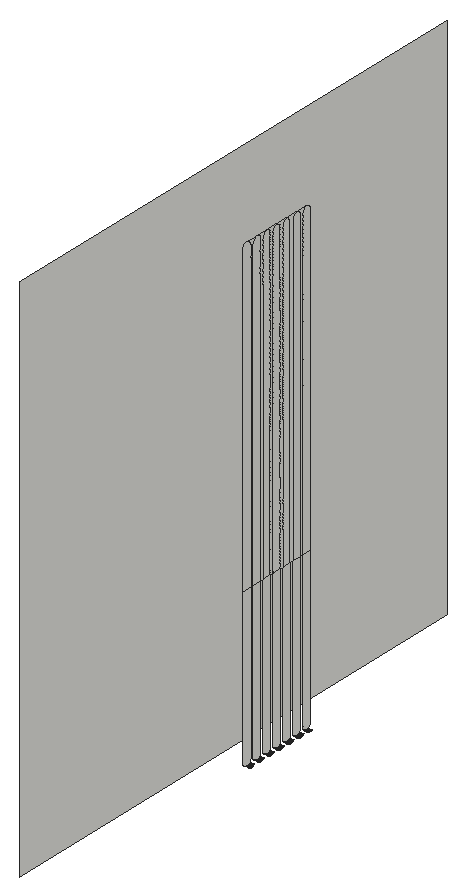
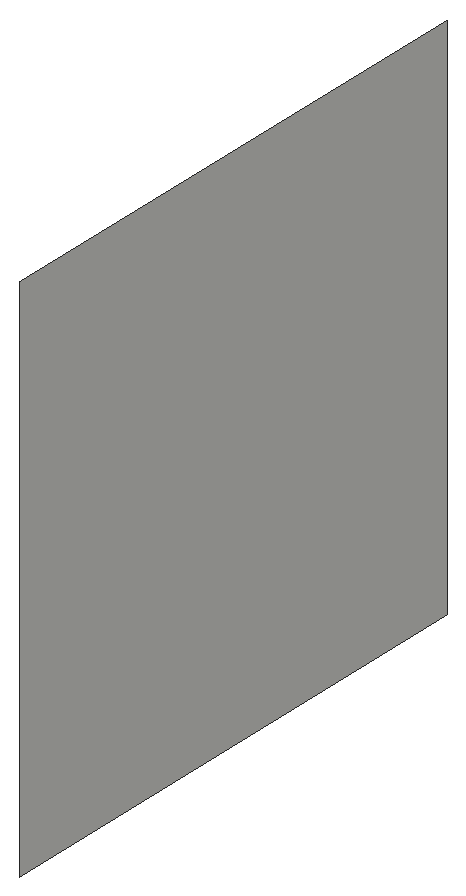
# SketchUp Ruby script. Lengths in inches.
U = 1.inch
M = Sketchup.active_model
def pt(a) = Geom::Point3d.new(a.map { |v| v * U })
def face(e, loops, mat)
  f = e.add_face(loops[0].map { |a| pt(a) })
  loops[1..].each { |l| e.add_face(l.map { |a| pt(a) }).erase! }
  f.material = f.back_material = mat if mat
  f
end
# faces: each face lists its corners as indices into pts; further lists are holes
def faces(e, pts, list, mat = nil) = list.each { |f| face(e, (f[0].is_a?(Array) ? f : [f]).map { |l| l.map { |i| pts[i] } }, mat) }
# xy, xz, yz: faces in a plane at the given z, y or x. An outline is a flat list of corners, or four numbers for a rectangle; further outlines are holes
def ring(l) = l.size == 4 ? [[l[0], l[1]], [l[2], l[1]], [l[2], l[3]], [l[0], l[3]]] : l.each_slice(2).to_a
def flat(e, list, mat, &to3) = list.each { |f| face(e, (f[0].is_a?(Array) ? f : [f]).map { |l| ring(l).map { |u, v| to3.(u, v) } }, mat) }
def xy(e, z, list, mat = nil) = flat(e, list, mat) { |x, y| [x, y, z] }
def xz(e, y, list, mat = nil) = flat(e, list, mat) { |x, z| [x, y, z] }
def yz(e, x, list, mat = nil) = flat(e, list, mat) { |y, z| [x, y, z] }
def lines(e, pts, list) = list.each { |a, b| e.add_line(pt(pts[a]), pt(pts[b])) }
# prism: a flat outline (further loops are holes) pulled along v
def prism(e, loops, v, mat = nil)
  f = face(e, loops, mat); d = Geom::Vector3d.new(v.map { |x| x * U })
  f.pushpull(f.normal.samedirection?(d) ? d.length : -d.length)
end
def box(e, o, s, mat = nil) = prism(e, [[o, [o[0] + s[0], o[1], o[2]], [o[0] + s[0], o[1] + s[1], o[2]], [o[0], o[1] + s[1], o[2]]]], [0, 0, s[2]], mat)
def at(x, y, z, deg = 0) = Geom::Transformation.translation(pt([x, y, z])) * Geom::Transformation.rotation(ORIGIN, Z_AXIS, deg.degrees)
def axes(o, x, y, z) = Geom::Transformation.new([*x, 0, *y, 0, *z, 0, *pt(o).to_a, 1])
def part(name) = M.definitions.add(name)
# library, detail: a bought-in or finely detailed component or shape, given as its bounding box
def library(name, o, s) = part(name).tap { |d| box(d.entities, o, s) }
def detail(e, o, s) = box(e.add_group.entities, o, s)
def put(e, d, t, mat = nil) = e.add_instance(d, t).tap { |i| i.material = mat if mat }
def group(e, t, mat = nil) = e.add_group.tap { |g| g.transformation = t; g.material = mat if mat }.entities
root = M.entities
yz(root,0,[[0,0,120,120]])
yz(root,9,[[52.509,2.396,52.567,2.398,52.624,2.403,52.681,2.41,52.737,2.421,52.792,2.435,52.847,2.452,52.901,2.473,52.954,2.495,53.005,2.521,53.054,2.55,53.103,2.581,53.149,2.615,53.193,2.651,53.235,2.69,53.276,2.731,53.313,2.774,53.349,2.82,53.381,2.867,53.412,2.915,53.439,2.966,53.464,3.018,53.486,3.071,53.504,3.125,53.52,3.18,53.533,3.236,53.543,3.292,53.55,3.363,53.55,38,51.468,38,51.468,3.363,51.476,3.292,51.486,3.236,51.498,3.18,51.514,3.125,51.533,3.071,51.555,3.018,51.579,2.966,51.607,2.915,51.637,2.867,51.67,2.82,51.705,2.774,51.743,2.731,51.783,2.69,51.825,2.651,51.87,2.615,51.916,2.581,51.964,2.55,52.014,2.521,52.065,2.495,52.118,2.473,52.171,2.452,52.226,2.435,52.282,2.421,52.338,2.41,52.395,2.403,52.452,2.398],[55.297,2.396,55.354,2.398,55.411,2.403,55.468,2.41,55.524,2.421,55.58,2.435,55.635,2.452,55.688,2.473,55.741,2.495,55.792,2.521,55.842,2.55,55.89,2.581,55.936,2.615,55.981,2.651,56.023,2.69,56.063,2.731,56.101,2.774,56.136,2.82,56.169,2.867,56.199,2.915,56.227,2.966,56.251,3.018,56.273,3.071,56.292,3.125,56.308,3.18,56.32,3.236,56.33,3.292,56.338,3.363,56.338,38,54.256,38,54.256,3.363,54.263,3.292,54.273,3.236,54.286,3.18,54.302,3.125,54.32,3.071,54.342,3.018,54.367,2.966,54.394,2.915,54.425,2.867,54.457,2.82,54.493,2.774,54.53,2.731,54.571,2.69,54.613,2.651,54.657,2.615,54.703,2.581,54.752,2.55,54.801,2.521,54.852,2.495,54.905,2.473,54.959,2.452,55.014,2.435,55.069,2.421,55.125,2.41,55.182,2.403,55.239,2.398],[58.084,2.396,58.142,2.398,58.199,2.403,58.256,2.41,58.312,2.421,58.367,2.435,58.422,2.452,58.476,2.473,58.529,2.495,58.58,2.521,58.629,2.55,58.678,2.581,58.724,2.615,58.768,2.651,58.81,2.69,58.851,2.731,58.888,2.774,58.924,2.82,58.956,2.867,58.987,2.915,59.014,2.966,59.039,3.018,59.061,3.071,59.079,3.125,59.095,3.18,59.108,3.236,59.118,3.292,59.125,3.363,59.125,38,57.043,38,57.043,3.363,57.051,3.292,57.061,3.236,57.073,3.18,57.089,3.125,57.108,3.071,57.13,3.018,57.154,2.966,57.182,2.915,57.212,2.867,57.245,2.82,57.28,2.774,57.318,2.731,57.358,2.69,57.4,2.651,57.445,2.615,57.491,2.581,57.539,2.55,57.589,2.521,57.64,2.495,57.693,2.473,57.746,2.452,57.801,2.435,57.857,2.421,57.913,2.41,57.97,2.403,58.027,2.398],[60.872,2.396,60.929,2.398,60.986,2.403,61.043,2.41,61.099,2.421,61.155,2.435,61.21,2.452,61.263,2.473,61.316,2.495,61.367,2.521,61.417,2.55,61.465,2.581,61.511,2.615,61.556,2.651,61.598,2.69,61.638,2.731,61.676,2.774,61.711,2.82,61.744,2.867,61.774,2.915,61.802,2.966,61.826,3.018,61.848,3.071,61.867,3.125,61.883,3.18,61.895,3.236,61.905,3.292,61.912,3.363,61.912,38,59.831,38,59.831,3.363,59.838,3.292,59.848,3.236,59.861,3.18,59.877,3.125,59.895,3.071,59.917,3.018,59.942,2.966,59.969,2.915,60,2.867,60.032,2.82,60.068,2.774,60.105,2.731,60.146,2.69,60.188,2.651,60.232,2.615,60.278,2.581,60.327,2.55,60.376,2.521,60.427,2.495,60.48,2.473,60.534,2.452,60.589,2.435,60.644,2.421,60.7,2.41,60.757,2.403,60.814,2.398],[63.659,2.396,63.717,2.398,63.774,2.403,63.831,2.41,63.887,2.421,63.942,2.435,63.997,2.452,64.051,2.473,64.104,2.495,64.155,2.521,64.204,2.55,64.253,2.581,64.299,2.615,64.343,2.651,64.385,2.69,64.426,2.731,64.463,2.774,64.499,2.82,64.531,2.867,64.562,2.915,64.589,2.966,64.614,3.018,64.636,3.071,64.654,3.125,64.67,3.18,64.683,3.236,64.693,3.292,64.7,3.363,64.7,38,62.618,38,62.618,3.363,62.626,3.292,62.636,3.236,62.648,3.18,62.664,3.125,62.683,3.071,62.705,3.018,62.729,2.966,62.757,2.915,62.787,2.867,62.82,2.82,62.855,2.774,62.893,2.731,62.933,2.69,62.975,2.651,63.02,2.615,63.066,2.581,63.114,2.55,63.164,2.521,63.215,2.495,63.268,2.473,63.321,2.452,63.376,2.435,63.432,2.421,63.488,2.41,63.545,2.403,63.602,2.398],
  [66.447,2.396,66.504,2.398,66.561,2.403,66.618,2.41,66.674,2.421,66.73,2.435,66.785,2.452,66.838,2.473,66.891,2.495,66.942,2.521,66.992,2.55,67.04,2.581,67.086,2.615,67.131,2.651,67.173,2.69,67.213,2.731,67.251,2.774,67.286,2.82,67.319,2.867,67.349,2.915,67.377,2.966,67.401,3.018,67.423,3.071,67.442,3.125,67.458,3.18,67.47,3.236,67.48,3.292,67.487,3.363,67.487,38,65.406,38,65.406,3.363,65.413,3.292,65.423,3.236,65.436,3.18,65.452,3.125,65.47,3.071,65.492,3.018,65.517,2.966,65.544,2.915,65.575,2.867,65.607,2.82,65.643,2.774,65.68,2.731,65.721,2.69,65.763,2.651,65.807,2.615,65.853,2.581,65.902,2.55,65.951,2.521,66.002,2.495,66.055,2.473,66.109,2.452,66.164,2.435,66.219,2.421,66.275,2.41,66.332,2.403,66.389,2.398],[69.234,2.396,69.292,2.398,69.349,2.403,69.406,2.41,69.462,2.421,69.517,2.435,69.572,2.452,69.626,2.473,69.679,2.495,69.73,2.521,69.779,2.55,69.828,2.581,69.874,2.615,69.918,2.651,69.96,2.69,70.001,2.731,70.038,2.774,70.074,2.82,70.106,2.867,70.137,2.915,70.164,2.966,70.189,3.018,70.211,3.071,70.229,3.125,70.245,3.18,70.258,3.236,70.268,3.292,70.275,3.363,70.275,38,68.193,38,68.193,3.363,68.201,3.292,68.211,3.236,68.223,3.18,68.239,3.125,68.258,3.071,68.28,3.018,68.304,2.966,68.332,2.915,68.362,2.867,68.395,2.82,68.43,2.774,68.468,2.731,68.508,2.69,68.55,2.651,68.595,2.615,68.641,2.581,68.689,2.55,68.739,2.521,68.79,2.495,68.843,2.473,68.896,2.452,68.951,2.435,69.007,2.421,69.063,2.41,69.12,2.403,69.177,2.398],[53.55,3.363,53.553,3.407,53.553,3.464,53.55,3.521],[54.256,3.363,54.256,3.521,54.253,3.464,54.253,3.407],[56.338,3.363,56.34,3.407,56.34,3.464,56.338,3.521],
  [57.043,3.363,57.043,3.521,57.041,3.464,57.041,3.407],[59.125,3.363,59.128,3.407,59.128,3.464,59.125,3.521],[59.831,3.363,59.831,3.521,59.828,3.464,59.828,3.407],[61.912,3.363,61.915,3.407,61.915,3.464,61.912,3.521],[62.618,3.363,62.618,3.521,62.616,3.464,62.616,3.407],
  [64.7,3.363,64.703,3.407,64.703,3.464,64.7,3.521],[65.406,3.363,65.406,3.521,65.403,3.464,65.403,3.407],[67.487,3.363,67.49,3.407,67.49,3.464,67.487,3.521],[68.193,3.363,68.193,3.521,68.191,3.464,68.191,3.407],[51.468,38,53.55,38,53.55,106.961,53.549,107.015,53.544,107.069,53.537,107.123,53.527,107.177,53.515,107.23,53.499,107.282,53.481,107.334,53.46,107.384,53.437,107.433,53.411,107.481,53.382,107.528,53.351,107.572,53.318,107.616,53.283,107.657,53.245,107.697,53.206,107.734,53.164,107.769,53.121,107.803,53.076,107.834,53.03,107.862,52.982,107.888,52.933,107.911,52.882,107.932,52.831,107.95,52.779,107.966,52.726,107.979,52.672,107.989,52.618,107.996,52.564,108,52.455,108,52.4,107.996,52.346,107.989,52.293,107.979,52.24,107.966,52.1875,107.95,52.136,107.932,52.086,107.911,52.037,107.888,51.989,107.862,51.942,107.834,51.898,107.803,51.854,107.769,51.813,107.734,51.773,107.697,51.736,107.657,51.7,107.616,51.667,107.572,51.636,107.528,51.608,107.481,51.582,107.433,51.558,107.384,51.538,107.334,51.519,107.282,51.504,107.23,51.491,107.177,51.481,107.123,51.474,107.069,51.47,107.015,51.468,106.961],
  [53.55,38,54.256,38,54.256,106.961,54.257,107.015,54.262,107.069,54.269,107.123,54.279,107.177,54.291,107.23,54.307,107.282,54.325,107.334,54.346,107.384,54.369,107.433,54.395,107.481,54.424,107.528,54.455,107.572,54.488,107.616,54.523,107.657,54.561,107.697,54.6,107.734,54.642,107.769,54.685,107.803,54.73,107.834,54.776,107.862,54.824,107.888,54.873,107.911,54.924,107.932,54.975,107.95,55.027,107.966,55.08,107.979,55.134,107.989,55.188,107.996,55.242,108,52.564,108,52.618,107.996,52.672,107.989,52.726,107.979,52.779,107.966,52.831,107.95,52.882,107.932,52.933,107.911,52.982,107.888,53.03,107.862,53.076,107.834,53.121,107.803,53.164,107.769,53.206,107.734,53.245,107.697,53.283,107.657,53.318,107.616,53.351,107.572,53.382,107.528,53.411,107.481,53.437,107.433,53.46,107.384,53.481,107.334,53.499,107.282,53.515,107.23,53.527,107.177,53.537,107.123,53.544,107.069,53.549,107.015,53.55,106.961],[54.256,38,56.338,38,56.338,106.961,56.336,107.015,56.332,107.069,56.325,107.123,56.315,107.177,56.302,107.23,56.287,107.282,56.268,107.334,56.248,107.384,56.224,107.433,56.198,107.481,56.17,107.528,56.139,107.572,56.106,107.616,56.07,107.657,56.033,107.697,55.993,107.734,55.952,107.769,55.908,107.803,55.864,107.834,55.817,107.862,55.769,107.888,55.72,107.911,55.67,107.932,55.618,107.95,55.566,107.966,55.513,107.979,55.46,107.989,55.406,107.996,55.351,108,55.242,108,55.188,107.996,55.134,107.989,55.08,107.979,55.027,107.966,54.975,107.95,54.924,107.932,54.873,107.911,54.824,107.888,54.776,107.862,54.73,107.834,54.685,107.803,54.642,107.769,54.6,107.734,54.561,107.697,54.523,107.657,54.488,107.616,54.455,107.572,54.424,107.528,54.395,107.481,54.369,107.433,54.346,107.384,54.325,107.334,54.307,107.282,54.291,107.23,54.279,107.177,54.269,107.123,54.262,107.069,54.257,107.015,54.256,106.961],[56.338,38,57.043,38,57.043,106.961,57.045,107.015,57.049,107.069,57.056,107.123,57.066,107.177,57.079,107.23,57.094,107.282,57.113,107.334,57.133,107.384,57.157,107.433,57.183,107.481,57.211,107.528,57.242,107.572,57.275,107.616,57.311,107.657,57.348,107.697,57.388,107.734,57.429,107.769,57.473,107.803,57.517,107.834,57.564,107.862,57.612,107.888,57.661,107.911,57.711,107.932,57.763,107.95,57.815,107.966,57.868,107.979,57.921,107.989,57.975,107.996,58.03,108,55.351,108,55.406,107.996,55.46,107.989,55.513,107.979,55.566,107.966,55.618,107.95,55.67,107.932,55.72,107.911,55.769,107.888,55.817,107.862,55.864,107.834,55.908,107.803,55.952,107.769,55.993,107.734,56.033,107.697,56.07,107.657,56.106,107.616,56.139,107.572,56.17,107.528,56.198,107.481,56.224,107.433,56.248,107.384,56.268,107.334,56.287,107.282,56.302,107.23,56.315,107.177,56.325,107.123,56.332,107.069,56.336,107.015,56.338,106.961],[57.043,38,59.125,38,59.125,106.961,59.124,107.015,59.119,107.069,59.112,107.123,59.102,107.177,59.09,107.23,59.074,107.282,59.056,107.334,59.035,107.384,59.012,107.433,58.986,107.481,58.957,107.528,58.926,107.572,58.893,107.616,58.858,107.657,58.82,107.697,58.781,107.734,58.739,107.769,58.696,107.803,58.651,107.834,58.605,107.862,58.557,107.888,58.508,107.911,58.457,107.932,58.406,107.95,58.354,107.966,58.301,107.979,58.247,107.989,58.193,107.996,58.139,108,58.03,108,57.975,107.996,57.921,107.989,57.868,107.979,57.815,107.966,57.763,107.95,57.711,107.932,57.661,107.911,57.612,107.888,57.564,107.862,57.517,107.834,57.473,107.803,57.429,107.769,57.388,107.734,57.348,107.697,57.311,107.657,57.275,107.616,57.242,107.572,57.211,107.528,57.183,107.481,57.157,107.433,57.133,107.384,57.113,107.334,57.094,107.282,57.079,107.23,57.066,107.177,57.056,107.123,57.049,107.069,57.045,107.015,57.043,106.961],[59.125,38,59.831,38,59.831,106.961,59.832,107.015,59.837,107.069,59.844,107.123,59.854,107.177,59.866,107.23,59.882,107.282,59.9,107.334,59.921,107.384,59.944,107.433,59.97,107.481,59.999,107.528,60.03,107.572,60.063,107.616,60.098,107.657,60.136,107.697,60.175,107.734,60.217,107.769,60.26,107.803,60.305,107.834,60.351,107.862,60.399,107.888,60.448,107.911,60.499,107.932,60.55,107.95,60.602,107.966,60.655,107.979,60.709,107.989,60.763,107.996,60.817,108,58.139,108,58.193,107.996,58.247,107.989,58.301,107.979,58.354,107.966,58.406,107.95,58.457,107.932,58.508,107.911,58.557,107.888,58.605,107.862,58.651,107.834,58.696,107.803,58.739,107.769,58.781,107.734,58.82,107.697,58.858,107.657,58.893,107.616,58.926,107.572,58.957,107.528,58.986,107.481,59.012,107.433,59.035,107.384,59.056,107.334,59.074,107.282,59.09,107.23,59.102,107.177,59.112,107.123,59.119,107.069,59.124,107.015,59.125,106.961],
  [59.831,38,61.912,38,61.912,106.961,61.911,107.015,61.907,107.069,61.9,107.123,61.89,107.177,61.877,107.23,61.862,107.282,61.843,107.334,61.823,107.384,61.799,107.433,61.773,107.481,61.745,107.528,61.714,107.572,61.681,107.616,61.645,107.657,61.608,107.697,61.568,107.734,61.527,107.769,61.483,107.803,61.439,107.834,61.392,107.862,61.344,107.888,61.295,107.911,61.245,107.932,61.193,107.95,61.141,107.966,61.088,107.979,61.035,107.989,60.981,107.996,60.926,108,60.817,108,60.763,107.996,60.709,107.989,60.655,107.979,60.602,107.966,60.55,107.95,60.499,107.932,60.448,107.911,60.399,107.888,60.351,107.862,60.305,107.834,60.26,107.803,60.217,107.769,60.175,107.734,60.136,107.697,60.098,107.657,60.063,107.616,60.03,107.572,59.999,107.528,59.97,107.481,59.944,107.433,59.921,107.384,59.9,107.334,59.882,107.282,59.866,107.23,59.854,107.177,59.844,107.123,59.837,107.069,59.832,107.015,59.831,106.961],[61.912,38,62.618,38,62.618,106.961,62.62,107.015,62.624,107.069,62.631,107.123,62.641,107.177,62.654,107.23,62.669,107.282,62.6875,107.334,62.708,107.384,62.732,107.433,62.758,107.481,62.786,107.528,62.817,107.572,62.85,107.616,62.886,107.657,62.923,107.697,62.963,107.734,63.004,107.769,63.048,107.803,63.092,107.834,63.139,107.862,63.187,107.888,63.236,107.911,63.286,107.932,63.338,107.95,63.39,107.966,63.443,107.979,63.496,107.989,63.55,107.996,63.605,108,60.926,108,60.981,107.996,61.035,107.989,61.088,107.979,61.141,107.966,61.193,107.95,61.245,107.932,61.295,107.911,61.344,107.888,61.392,107.862,61.439,107.834,61.483,107.803,61.527,107.769,61.568,107.734,61.608,107.697,61.645,107.657,61.681,107.616,61.714,107.572,61.745,107.528,61.773,107.481,61.799,107.433,61.823,107.384,61.843,107.334,61.862,107.282,61.877,107.23,61.89,107.177,61.9,107.123,61.907,107.069,61.911,107.015,61.912,106.961],[62.618,38,64.7,38,64.7,106.961,64.699,107.015,64.694,107.069,64.687,107.123,64.677,107.177,64.665,107.23,64.649,107.282,64.631,107.334,64.61,107.384,64.587,107.433,64.561,107.481,64.532,107.528,64.501,107.572,64.468,107.616,64.433,107.657,64.395,107.697,64.356,107.734,64.314,107.769,64.271,107.803,64.226,107.834,64.18,107.862,64.132,107.888,64.083,107.911,64.032,107.932,63.981,107.95,63.929,107.966,63.876,107.979,63.822,107.989,63.768,107.996,63.714,108,63.605,108,63.55,107.996,63.496,107.989,63.443,107.979,63.39,107.966,63.338,107.95,63.286,107.932,63.236,107.911,63.187,107.888,63.139,107.862,63.092,107.834,63.048,107.803,63.004,107.769,62.963,107.734,62.923,107.697,62.886,107.657,62.85,107.616,62.817,107.572,62.786,107.528,62.758,107.481,62.732,107.433,62.708,107.384,62.6875,107.334,62.669,107.282,62.654,107.23,62.641,107.177,62.631,107.123,62.624,107.069,62.62,107.015,62.618,106.961],[64.7,38,65.406,38,65.406,106.961,65.407,107.015,65.412,107.069,65.419,107.123,65.429,107.177,65.441,107.23,65.457,107.282,65.475,107.334,65.496,107.384,65.519,107.433,65.545,107.481,65.574,107.528,65.605,107.572,65.638,107.616,65.673,107.657,65.711,107.697,65.75,107.734,65.792,107.769,65.835,107.803,65.88,107.834,65.926,107.862,65.974,107.888,66.023,107.911,66.074,107.932,66.125,107.95,66.177,107.966,66.23,107.979,66.284,107.989,66.338,107.996,66.392,108,63.714,108,63.768,107.996,63.822,107.989,63.876,107.979,63.929,107.966,63.981,107.95,64.032,107.932,64.083,107.911,64.132,107.888,64.18,107.862,64.226,107.834,64.271,107.803,64.314,107.769,64.356,107.734,64.395,107.697,64.433,107.657,64.468,107.616,64.501,107.572,64.532,107.528,64.561,107.481,64.587,107.433,64.61,107.384,64.631,107.334,64.649,107.282,64.665,107.23,64.677,107.177,64.687,107.123,64.694,107.069,64.699,107.015,64.7,106.961],[65.406,38,67.487,38,67.487,106.961,67.486,107.015,67.482,107.069,67.475,107.123,67.465,107.177,67.452,107.23,67.437,107.282,67.418,107.334,67.398,107.384,67.374,107.433,67.348,107.481,67.32,107.528,67.289,107.572,67.256,107.616,67.22,107.657,67.183,107.697,67.143,107.734,67.102,107.769,67.058,107.803,67.014,107.834,66.967,107.862,66.919,107.888,66.87,107.911,66.82,107.932,66.768,107.95,66.716,107.966,66.663,107.979,66.61,107.989,66.556,107.996,66.501,108,66.392,108,66.338,107.996,66.284,107.989,66.23,107.979,66.177,107.966,66.125,107.95,66.074,107.932,66.023,107.911,65.974,107.888,65.926,107.862,65.88,107.834,65.835,107.803,65.792,107.769,65.75,107.734,65.711,107.697,65.673,107.657,65.638,107.616,65.605,107.572,65.574,107.528,65.545,107.481,65.519,107.433,65.496,107.384,65.475,107.334,65.457,107.282,65.441,107.23,65.429,107.177,65.419,107.123,65.412,107.069,65.407,107.015,65.406,106.961],
  [67.487,38,68.193,38,68.193,106.961,68.195,107.015,68.199,107.069,68.206,107.123,68.216,107.177,68.229,107.23,68.244,107.282,68.263,107.334,68.283,107.384,68.307,107.433,68.333,107.481,68.361,107.528,68.392,107.572,68.425,107.616,68.461,107.657,68.498,107.697,68.538,107.734,68.579,107.769,68.623,107.803,68.667,107.834,68.714,107.862,68.762,107.888,68.811,107.911,68.861,107.932,68.913,107.95,68.965,107.966,69.018,107.979,69.071,107.989,69.125,107.996,69.18,108,66.501,108,66.556,107.996,66.61,107.989,66.663,107.979,66.716,107.966,66.768,107.95,66.82,107.932,66.87,107.911,66.919,107.888,66.967,107.862,67.014,107.834,67.058,107.803,67.102,107.769,67.143,107.734,67.183,107.697,67.22,107.657,67.256,107.616,67.289,107.572,67.32,107.528,67.348,107.481,67.374,107.433,67.398,107.384,67.418,107.334,67.437,107.282,67.452,107.23,67.465,107.177,67.475,107.123,67.482,107.069,67.486,107.015,67.487,106.961],[68.193,38,70.275,38,70.275,106.961,70.274,107.015,70.269,107.069,70.262,107.123,70.252,107.177,70.24,107.23,70.224,107.282,70.206,107.334,70.185,107.384,70.162,107.433,70.136,107.481,70.107,107.528,70.076,107.572,70.043,107.616,70.008,107.657,69.97,107.697,69.931,107.734,69.889,107.769,69.846,107.803,69.801,107.834,69.755,107.862,69.707,107.888,69.658,107.911,69.607,107.932,69.556,107.95,69.504,107.966,69.451,107.979,69.397,107.989,69.343,107.996,69.289,108,69.18,108,69.125,107.996,69.071,107.989,69.018,107.979,68.965,107.966,68.913,107.95,68.861,107.932,68.811,107.911,68.762,107.888,68.714,107.862,68.667,107.834,68.623,107.803,68.579,107.769,68.538,107.734,68.498,107.697,68.461,107.657,68.425,107.616,68.392,107.572,68.361,107.528,68.333,107.481,68.307,107.433,68.283,107.384,68.263,107.334,68.244,107.282,68.229,107.23,68.216,107.177,68.206,107.123,68.199,107.069,68.195,107.015,68.193,106.961]])
p = [[9,52.171,2.452],[9,52.226,2.435],[10,52.226,2.435],[10,52.171,2.452],[9,52.282,2.421],[10,52.282,2.421],
  [9,52.338,2.41],[10,52.338,2.41],[9,52.395,2.403],[10,52.395,2.403],[9,52.452,2.398],[10,52.452,2.398],
  [9,52.509,2.396],[10,52.509,2.396],[9,52.567,2.398],[10,52.567,2.398],[9,52.624,2.403],[10,52.624,2.403],
  [9,52.681,2.41],[10,52.681,2.41],[9,52.737,2.421],[10,52.737,2.421],[9,52.792,2.435],[10,52.792,2.435],
  [9,52.847,2.452],[10,52.847,2.452],[9,54.959,2.452],[9,55.014,2.435],[10,55.014,2.435],[10,54.959,2.452],
  [9,55.069,2.421],[10,55.069,2.421],[9,55.125,2.41],[10,55.125,2.41],[9,55.182,2.403],[10,55.182,2.403],
  [9,55.239,2.398],[10,55.239,2.398],[9,55.297,2.396],[10,55.297,2.396],[9,55.354,2.398],[10,55.354,2.398],
  [9,55.411,2.403],[10,55.411,2.403],[9,55.468,2.41],[10,55.468,2.41],[9,55.524,2.421],[10,55.524,2.421],
  [9,55.58,2.435],[10,55.58,2.435],[9,55.635,2.452],[10,55.635,2.452],[9,57.746,2.452],[9,57.801,2.435],
  [10,57.801,2.435],[10,57.746,2.452],[9,57.857,2.421],[10,57.857,2.421],[9,57.913,2.41],[10,57.913,2.41],
  [9,57.97,2.403],[10,57.97,2.403],[9,58.027,2.398],[10,58.027,2.398],[9,58.084,2.396],[10,58.084,2.396],
  [9,58.142,2.398],[10,58.142,2.398],[9,58.199,2.403],[10,58.199,2.403],[9,58.256,2.41],[10,58.256,2.41],
  [9,58.312,2.421],[10,58.312,2.421],[9,58.367,2.435],[10,58.367,2.435],[9,58.422,2.452],[10,58.422,2.452],
  [9,60.534,2.452],[9,60.589,2.435],[10,60.589,2.435],[10,60.534,2.452],[9,60.644,2.421],[10,60.644,2.421],
  [9,60.7,2.41],[10,60.7,2.41],[9,60.757,2.403],[10,60.757,2.403],[9,60.814,2.398],[10,60.814,2.398],
  [9,60.872,2.396],[10,60.872,2.396],[9,60.929,2.398],[10,60.929,2.398],[9,60.986,2.403],[10,60.986,2.403],
  [9,61.043,2.41],[10,61.043,2.41],[9,61.099,2.421],[10,61.099,2.421],[9,61.155,2.435],[10,61.155,2.435],
  [9,61.21,2.452],[10,61.21,2.452],[9,63.321,2.452],[9,63.376,2.435],[10,63.376,2.435],[10,63.321,2.452],
  [9,63.432,2.421],[10,63.432,2.421],[9,63.488,2.41],[10,63.488,2.41],[9,63.545,2.403],[10,63.545,2.403],
  [9,63.602,2.398],[10,63.602,2.398],[9,63.659,2.396],[10,63.659,2.396],[9,63.717,2.398],[10,63.717,2.398],
  [9,63.774,2.403],[10,63.774,2.403],[9,63.831,2.41],[10,63.831,2.41],[9,63.887,2.421],[10,63.887,2.421],
  [9,63.942,2.435],[10,63.942,2.435],[9,63.997,2.452],[10,63.997,2.452],[9,66.109,2.452],[9,66.164,2.435],
  [10,66.164,2.435],[10,66.109,2.452],[9,66.219,2.421],[10,66.219,2.421],[9,66.275,2.41],[10,66.275,2.41],
  [9,66.332,2.403],[10,66.332,2.403],[9,66.389,2.398],[10,66.389,2.398],[9,66.447,2.396],[10,66.447,2.396],
  [9,66.504,2.398],[10,66.504,2.398],[9,66.561,2.403],[10,66.561,2.403],[9,66.618,2.41],[10,66.618,2.41],
  [9,66.674,2.421],[10,66.674,2.421],[9,66.73,2.435],[10,66.73,2.435],[9,66.785,2.452],[10,66.785,2.452],
  [9,68.896,2.452],[9,68.951,2.435],[10,68.951,2.435],[10,68.896,2.452],[9,69.007,2.421],[10,69.007,2.421],
  [9,69.063,2.41],[10,69.063,2.41],[9,69.12,2.403],[10,69.12,2.403],[9,69.177,2.398],[10,69.177,2.398],
  [9,69.234,2.396],[10,69.234,2.396],[9,69.292,2.398],[10,69.292,2.398],[9,69.349,2.403],[10,69.349,2.403],
  [9,69.406,2.41],[10,69.406,2.41],[9,69.462,2.421],[10,69.462,2.421],[9,69.517,2.435],[10,69.517,2.435],
  [9,69.572,2.452],[10,69.572,2.452],[9,52.014,2.521],[9,52.065,2.495],[10,52.065,2.495],[10,52.014,2.521],
  [9,52.118,2.473],[10,52.118,2.473],[9,52.901,2.473],[10,52.901,2.473],[9,52.954,2.495],[10,52.954,2.495],
  [9,53.005,2.521],[10,53.005,2.521],[9,53.054,2.55],[10,53.054,2.55],[9,53.103,2.581],[10,53.103,2.581],
  [9,54.703,2.581],[9,54.752,2.55],[10,54.752,2.55],[10,54.703,2.581],[9,54.801,2.521],[10,54.801,2.521],
  [9,54.852,2.495],[10,54.852,2.495],[9,54.905,2.473],[10,54.905,2.473],[9,55.688,2.473],[10,55.688,2.473],
  [9,55.741,2.495],[10,55.741,2.495],[9,55.792,2.521],[10,55.792,2.521],[9,55.842,2.55],[10,55.842,2.55],
  [9,55.89,2.581],[10,55.89,2.581],[9,57.491,2.581],[9,57.539,2.55],[10,57.539,2.55],[10,57.491,2.581],
  [9,57.589,2.521],[10,57.589,2.521],[9,57.64,2.495],[10,57.64,2.495],[9,57.693,2.473],[10,57.693,2.473],
  [9,58.476,2.473],[10,58.476,2.473],[9,58.529,2.495],[10,58.529,2.495],[9,58.58,2.521],[10,58.58,2.521],
  [9,58.629,2.55],[10,58.629,2.55],[9,58.678,2.581],[10,58.678,2.581],[9,60.278,2.581],[9,60.327,2.55],
  [10,60.327,2.55],[10,60.278,2.581],[9,60.376,2.521],[10,60.376,2.521],[9,60.427,2.495],[10,60.427,2.495],
  [9,60.48,2.473],[10,60.48,2.473],[9,61.263,2.473],[10,61.263,2.473],[9,61.316,2.495],[10,61.316,2.495],
  [9,61.367,2.521],[10,61.367,2.521],[9,61.417,2.55],[10,61.417,2.55],[9,61.465,2.581],[10,61.465,2.581],
  [9,63.066,2.581],[9,63.114,2.55],[10,63.114,2.55],[10,63.066,2.581],[9,63.164,2.521],[10,63.164,2.521],
  [9,63.215,2.495],[10,63.215,2.495],[9,63.268,2.473],[10,63.268,2.473],[9,64.051,2.473],[10,64.051,2.473],
  [9,64.104,2.495],[10,64.104,2.495],[9,64.155,2.521],[10,64.155,2.521],[9,64.204,2.55],[10,64.204,2.55],
  [9,64.253,2.581],[10,64.253,2.581],[9,65.853,2.581],[9,65.902,2.55],[10,65.902,2.55],[10,65.853,2.581],
  [9,65.951,2.521],[10,65.951,2.521],[9,66.002,2.495],[10,66.002,2.495],[9,66.055,2.473],[10,66.055,2.473],
  [9,66.838,2.473],[10,66.838,2.473],[9,66.891,2.495],[10,66.891,2.495],[9,66.942,2.521],[10,66.942,2.521],
  [9,66.992,2.55],[10,66.992,2.55],[9,67.04,2.581],[10,67.04,2.581],[9,68.641,2.581],[9,68.689,2.55],
  [10,68.689,2.55],[10,68.641,2.581],[9,68.739,2.521],[10,68.739,2.521],[9,68.79,2.495],[10,68.79,2.495],
  [9,68.843,2.473],[10,68.843,2.473],[9,53.149,2.615],[10,53.149,2.615],[9,53.193,2.651],[10,53.193,2.651],
  [9,54.613,2.651],[9,54.657,2.615],[10,54.657,2.615],[10,54.613,2.651],[9,55.936,2.615],[10,55.936,2.615],
  [9,55.981,2.651],[10,55.981,2.651],[9,57.4,2.651],[9,57.445,2.615],[10,57.445,2.615],[10,57.4,2.651],
  [9,58.724,2.615],[10,58.724,2.615],[9,58.768,2.651],[10,58.768,2.651],[9,60.188,2.651],[9,60.232,2.615],
  [10,60.232,2.615],[10,60.188,2.651],[9,61.511,2.615],[10,61.511,2.615],[9,61.556,2.651],[10,61.556,2.651],
  [9,62.975,2.651],[9,63.02,2.615],[10,63.02,2.615],[10,62.975,2.651],[9,64.299,2.615],[10,64.299,2.615],
  [9,64.343,2.651],[10,64.343,2.651],[9,65.763,2.651],[9,65.807,2.615],[10,65.807,2.615],[10,65.763,2.651],
  [9,67.086,2.615],[10,67.086,2.615],[9,67.131,2.651],[10,67.131,2.651],[9,68.55,2.651],[9,68.595,2.615],
  [10,68.595,2.615],[10,68.55,2.651],[9,53.235,2.69],[10,53.235,2.69],[9,53.276,2.731],[10,53.276,2.731],
  [9,54.571,2.69],[10,54.571,2.69],[9,56.023,2.69],[10,56.023,2.69],[9,56.063,2.731],[10,56.063,2.731],
  [9,57.358,2.69],[10,57.358,2.69],[9,58.81,2.69],[10,58.81,2.69],[9,58.851,2.731],[10,58.851,2.731],
  [9,60.105,2.731],[9,60.146,2.69],[10,60.146,2.69],[10,60.105,2.731],[9,61.598,2.69],[10,61.598,2.69],
  [9,61.638,2.731],[10,61.638,2.731],[9,62.893,2.731],[9,62.933,2.69],[10,62.933,2.69],[10,62.893,2.731],
  [9,64.385,2.69],[10,64.385,2.69],[9,64.426,2.731],[10,64.426,2.731],[9,65.68,2.731],[9,65.721,2.69],
  [10,65.721,2.69],[10,65.68,2.731],[9,67.173,2.69],[10,67.173,2.69],[9,67.213,2.731],[10,67.213,2.731],
  [9,68.468,2.731],[9,68.508,2.69],[10,68.508,2.69],[10,68.468,2.731]]
faces(root,p,[[0,1,2,3],[1,4,5,2],[4,6,7,5],[6,8,9,7],[8,10,11,9],[10,12,13,11],[12,14,15,13],[14,16,17,15],
  [16,18,19,17],[18,20,21,19],[20,22,23,21],[22,24,25,23],[26,27,28,29],[27,30,31,28],[30,32,33,31],[32,34,35,33],
  [34,36,37,35],[36,38,39,37],[38,40,41,39],[40,42,43,41],[42,44,45,43],[44,46,47,45],[46,48,49,47],[48,50,51,49],
  [52,53,54,55],[53,56,57,54],[56,58,59,57],[58,60,61,59],[60,62,63,61],[62,64,65,63],[64,66,67,65],[66,68,69,67],
  [68,70,71,69],[70,72,73,71],[72,74,75,73],[74,76,77,75],[78,79,80,81],[79,82,83,80],[82,84,85,83],[84,86,87,85],
  [86,88,89,87],[88,90,91,89],[90,92,93,91],[92,94,95,93],[94,96,97,95],[96,98,99,97],[98,100,101,99],[100,102,103,101],
  [104,105,106,107],[105,108,109,106],[108,110,111,109],[110,112,113,111],[112,114,115,113],[114,116,117,115],[116,118,119,117],[118,120,121,119],
  [120,122,123,121],[122,124,125,123],[124,126,127,125],[126,128,129,127],[130,131,132,133],[131,134,135,132],[134,136,137,135],[136,138,139,137],
  [138,140,141,139],[140,142,143,141],[142,144,145,143],[144,146,147,145],[146,148,149,147],[148,150,151,149],[150,152,153,151],[152,154,155,153],
  [156,157,158,159],[157,160,161,158],[160,162,163,161],[162,164,165,163],[164,166,167,165],[166,168,169,167],[168,170,171,169],[170,172,173,171],
  [172,174,175,173],[174,176,177,175],[176,178,179,177],[178,180,181,179],[182,183,184,185],[183,186,187,184],[186,0,3,187],[24,188,189,25],
  [188,190,191,189],[190,192,193,191],[192,194,195,193],[194,196,197,195],[198,199,200,201],[199,202,203,200],[202,204,205,203],[204,206,207,205],
  [206,26,29,207],[50,208,209,51],[208,210,211,209],[210,212,213,211],[212,214,215,213],[214,216,217,215],[218,219,220,221],[219,222,223,220],
  [222,224,225,223],[224,226,227,225],[226,52,55,227],[76,228,229,77],[228,230,231,229],[230,232,233,231],[232,234,235,233],[234,236,237,235],
  [238,239,240,241],[239,242,243,240],[242,244,245,243],[244,246,247,245],[246,78,81,247],[102,248,249,103],[248,250,251,249],[250,252,253,251],
  [252,254,255,253],[254,256,257,255],[258,259,260,261],[259,262,263,260],[262,264,265,263],[264,266,267,265],[266,104,107,267],[128,268,269,129],
  [268,270,271,269],[270,272,273,271],[272,274,275,273],[274,276,277,275],[278,279,280,281],[279,282,283,280],[282,284,285,283],[284,286,287,285],
  [286,130,133,287],[154,288,289,155],[288,290,291,289],[290,292,293,291],[292,294,295,293],[294,296,297,295],[298,299,300,301],[299,302,303,300],
  [302,304,305,303],[304,306,307,305],[306,156,159,307],[196,308,309,197],[308,310,311,309],[312,313,314,315],[313,198,201,314],[216,316,317,217],
  [316,318,319,317],[320,321,322,323],[321,218,221,322],[236,324,325,237],[324,326,327,325],[328,329,330,331],[329,238,241,330],[256,332,333,257],
  [332,334,335,333],[336,337,338,339],[337,258,261,338],[276,340,341,277],[340,342,343,341],[344,345,346,347],[345,278,281,346],[296,348,349,297],
  [348,350,351,349],[352,353,354,355],[353,298,301,354],[310,356,357,311],[356,358,359,357],[360,312,315,361],[318,362,363,319],[362,364,365,363],
  [366,320,323,367],[326,368,369,327],[368,370,371,369],[372,373,374,375],[373,328,331,374],[334,376,377,335],[376,378,379,377],[380,381,382,383],
  [381,336,339,382],[342,384,385,343],[384,386,387,385],[388,389,390,391],[389,344,347,390],[350,392,393,351],[392,394,395,393],[396,397,398,399],
  [397,352,355,398]])
